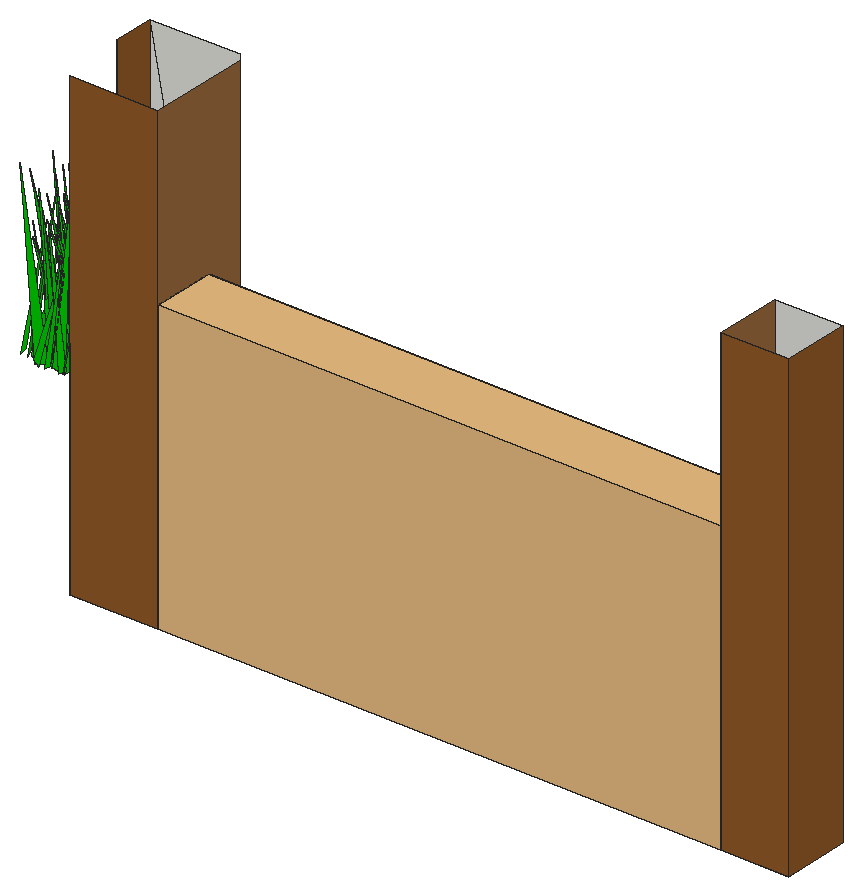
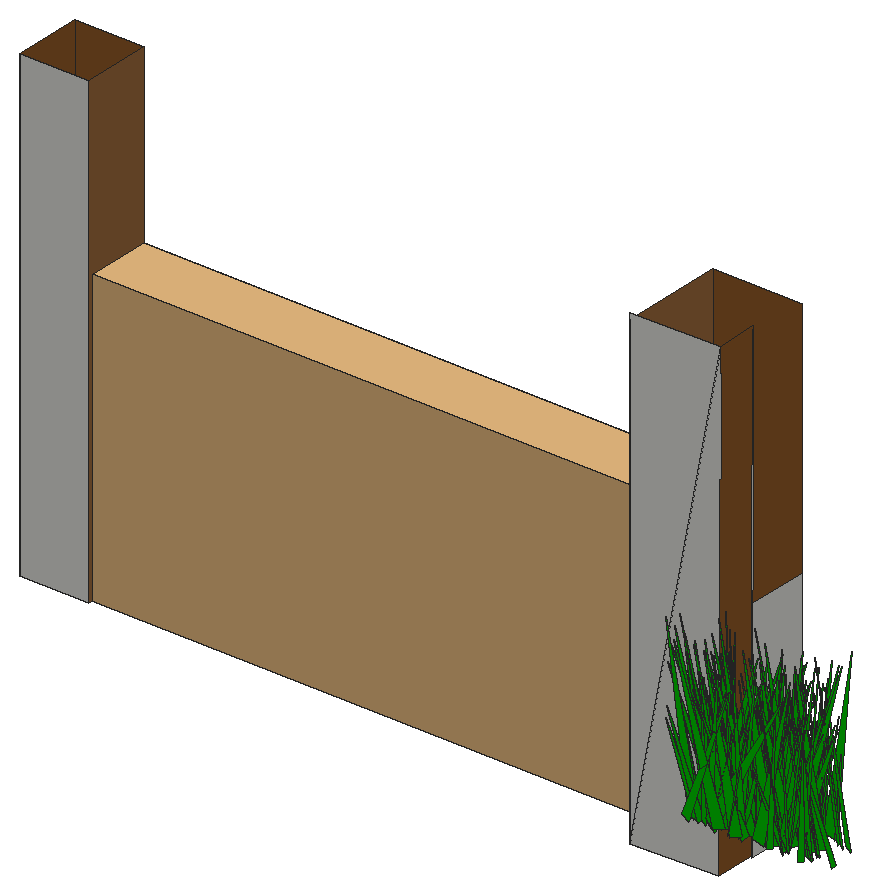
# SketchUp Ruby script. Lengths in inches.
U = 1.inch
M = Sketchup.active_model
def pt(a) = Geom::Point3d.new(a.map { |v| v * U })
def face(e, loops, mat)
  f = e.add_face(loops[0].map { |a| pt(a) })
  loops[1..].each { |l| e.add_face(l.map { |a| pt(a) }).erase! }
  f.material = f.back_material = mat if mat
  f
end
# faces: each face lists its corners as indices into pts; further lists are holes
def faces(e, pts, list, mat = nil) = list.each { |f| face(e, (f[0].is_a?(Array) ? f : [f]).map { |l| l.map { |i| pts[i] } }, mat) }
# xy, xz, yz: faces in a plane at the given z, y or x. An outline is a flat list of corners, or four numbers for a rectangle; further outlines are holes
def ring(l) = l.size == 4 ? [[l[0], l[1]], [l[2], l[1]], [l[2], l[3]], [l[0], l[3]]] : l.each_slice(2).to_a
def flat(e, list, mat, &to3) = list.each { |f| face(e, (f[0].is_a?(Array) ? f : [f]).map { |l| ring(l).map { |u, v| to3.(u, v) } }, mat) }
def xy(e, z, list, mat = nil) = flat(e, list, mat) { |x, y| [x, y, z] }
def xz(e, y, list, mat = nil) = flat(e, list, mat) { |x, z| [x, y, z] }
def yz(e, x, list, mat = nil) = flat(e, list, mat) { |y, z| [x, y, z] }
def lines(e, pts, list) = list.each { |a, b| e.add_line(pt(pts[a]), pt(pts[b])) }
# prism: a flat outline (further loops are holes) pulled along v
def prism(e, loops, v, mat = nil)
  f = face(e, loops, mat); d = Geom::Vector3d.new(v.map { |x| x * U })
  f.pushpull(f.normal.samedirection?(d) ? d.length : -d.length)
end
def box(e, o, s, mat = nil) = prism(e, [[o, [o[0] + s[0], o[1], o[2]], [o[0] + s[0], o[1] + s[1], o[2]], [o[0], o[1] + s[1], o[2]]]], [0, 0, s[2]], mat)
def at(x, y, z, deg = 0) = Geom::Transformation.translation(pt([x, y, z])) * Geom::Transformation.rotation(ORIGIN, Z_AXIS, deg.degrees)
def axes(o, x, y, z) = Geom::Transformation.new([*x, 0, *y, 0, *z, 0, *pt(o).to_a, 1])
def part(name) = M.definitions.add(name)
# library, detail: a bought-in or finely detailed component or shape, given as its bounding box
def library(name, o, s) = part(name).tap { |d| box(d.entities, o, s) }
def detail(e, o, s) = box(e.add_group.entities, o, s)
def put(e, d, t, mat = nil) = e.add_instance(d, t).tap { |i| i.material = mat if mat }
def group(e, t, mat = nil) = e.add_group.tap { |g| g.transformation = t; g.material = mat if mat }.entities
root = M.entities
M.materials.add("[Color G06]").color = [0, 204, 0]
M.materials.add("[Wood Floor Parquet]").color = [145, 89, 39]
M.materials.add("[Wood Floor]").color = [155, 105, 61]
c1 = part("fur_instance\#9")
p = [[0.8125,0,1.79],[0.67,-0.02,1.48],[0,-0.11,0],[0,0.11,0]]
faces(c1.entities,p,[[0,1,2,3]])
c2 = library("Modern+Gate+1",[0,0,0],[118.11,1.97,78.74])
xy(root,-6,[[121.48,2.125,121.48,8.54,121.67,8.29,121.67,12.5,130.61,12.75,130.61,2.125],[189.03,2.125,196.0625,9.15]])
xz(root,2.125,[[121.48,-6,130.61,42.1875],[189.03,-6,196.0625,42.0625]],"[Wood Floor Parquet]")
xz(root,9.15,[[189.03,-6,196.0625,42.0625]])
yz(root,121.48,[[2.125,-6,2.125,17.375,8.42,17.375,8.54,-6],[8.54,-6,8.54,17.375,8.42,17.375]])
yz(root,130.61,[[2.125,-6,12.75,42.1875]],"[Wood Floor]")
yz(root,189.03,[[2.125,-6,9.15,42.0625]],"[Wood Floor]")
yz(root,196.0625,[[2.125,-6,9.15,42.0625]],"[Wood Floor Parquet]")
p = [[121.67,8.29,-6],[121.48,8.54,-6],[121.48,8.42,17.375],[121.49,8.29,42.8125],[121.49,12.5,42.8125],[121.67,12.5,-6],
  [130.61,12.75,-6],[130.61,12.75,42.1875],[130.61,12.75,42.8125]]
faces(root,p,[[0,1,2,3],[5,4,6],[7,6,4,8]])
faces(root,p,[[3,4,5,0]],"[Wood Floor Parquet]")
put(root,c1,axes([107.31,16.14,4.28],[-2.23822,0.76515,2.70821],[5.77311,0.28435,1.42903],[-0.25036,-0.28356,8.74082]),"[Color G06]")
put(root,c1,axes([106.6875,16.22,4.28],[-2.84725,0.13927,0.80662],[0.78176,0.38789,-1.52926],[0.82315,0.11334,4.24241]),"[Color G06]")
put(root,c1,axes([106.91,20.07,4.28],[-5.58981,-0.32114,2.27191],[-2.05484,0.80404,1.76284],[1.84178,-0.07761,8.86202]),"[Color G06]")
put(root,c1,axes([104.89,16.85,4.28],[4.94685,-0.26614,0.07768],[-1.80121,-0.65722,-2.43716],[-0.63313,-0.20968,7.54053]),"[Color G06]")
put(root,c1,axes([103.96,19.85,4.28],[4.09901,0.34169,0.1307],[2.32033,-0.5329,-2.51227],[0.79237,-0.20708,6.68068]),"[Color G06]")
put(root,c1,axes([107.42,17.71,4.28],[-4.27879,-0.16322,0.91197],[-0.98771,0.58738,1.72486],[0.87568,-0.13501,6.40163]),"[Color G06]")
put(root,c1,axes([106.4,20,4.28],[2.27582,0.41603,0.63067],[2.88786,-0.3222,1.13794],[-0.85978,0.01899,5.49153]),"[Color G06]")
put(root,c1,axes([106.58,20.8,4.28],[-1.63991,-0.47873,0.1103],[-3.33168,0.22458,1.32609],[0.8317,-0.04431,5.5296]),"[Color G06]")
put(root,c1,axes([106,16.68,4.28],[4.25637,-0.02372,1.47172],[-0.34857,-0.59828,1.14406],[-0.93653,0.11486,6.26289]),"[Color G06]")
put(root,c1,axes([105.48,16.91,4.28],[5.82399,-0.07965,1.17242],[-0.36496,-0.7965,-2.16646],[-0.89913,-0.19262,8.47357]),"[Color G06]")
put(root,c1,axes([109.18,19.57,4.28],[-1.80742,-0.65842,1.18821],[-4.59181,0.20476,-2.5679],[-1.35702,0.18408,7.10652]),"[Color G06]")
put(root,c1,axes([106.25,19.24,4.28],[5.20739,0.12211,1.69695],[0.67046,-0.73455,1.47611],[-1.26745,0.11313,7.75282]),"[Color G06]")
put(root,c1,axes([106.3,19.02,4.28],[4.23846,0.37745,0.01663],[2.62839,-0.57459,1.77104],[-0.64692,0.13845,7.30465]),"[Color G06]")
put(root,c1,axes([108.73,19.88,4.28],[-5.82118,0.15488,1.36695],[0.79505,0.78927,-2.70996],[1.19917,0.22855,8.43237]),"[Color G06]")
put(root,c1,axes([109.85,17.24,4.28],[-4.58228,0.57529,1.07673],[4.15734,0.60686,2.27347],[-0.50588,-0.22385,8.93047]),"[Color G06]")
put(root,c1,axes([109.375,17.17,4.28],[-1.42676,-0.52227,1.51132],[-3.61847,0.12498,-2.66902],[-1.39885,0.20939,5.36261]),"[Color G06]")
put(root,c1,axes([108.07,16.57,4.28],[-4.25804,0.0751,1.83485],[-0.01705,0.56698,-2.75414],[1.34049,0.24576,5.79332]),"[Color G06]")
put(root,c1,axes([107.72,18.67,4.28],[-2.9836,-0.14143,1.40947],[-0.71691,0.42495,1.50868],[1.18496,-0.09902,4.46165]),"[Color G06]")
put(root,c1,axes([106.54,18.33,4.28],[-1.29654,0.83854,0.77196],[5.77566,0.19376,-2.50954],[1.75189,-0.01821,8.84482]),"[Color G06]")
put(root,c1,axes([108.1,16.31,4.28],[2.21507,0.47472,1.39601],[3.16348,-0.33517,1.88088],[-1.56671,-0.0056,5.77156]),"[Color G06]")
put(root,c1,axes([106.2,20.03,4.28],[4.19743,-0.1638,0.13344],[-1.13556,-0.57485,-1.27021],[-0.31341,-0.11086,6.38934]),"[Color G06]")
put(root,c1,axes([108.41,20.08,4.28],[-3.93748,-0.18116,1.02349],[-1.05205,0.53861,1.91099],[1.02468,-0.14315,5.89489]),"[Color G06]")
put(root,c1,axes([106.94,19.05,4.28],[0.48032,0.4754,1.33561],[3.45645,-0.03897,-1.18323],[0.68859,-0.136,5.00772]),"[Color G06]")
put(root,c1,axes([108.47,16.76,4.28],[1.50498,-0.80901,0.76967],[-5.64042,-0.22093,-2.041],[-1.45263,0.01969,8.72239]),"[Color G06]")
put(root,c1,axes([109.7,19.74,4.28],[-4.01086,-0.15859,0.02319],[-1.11322,0.54572,-1.35823],[-0.23335,0.12249,6.08103]),"[Color G06]")
put(root,c1,axes([109.2,19.4,4.28],[-2.44575,-0.30222,0.51286],[-2.16748,0.32156,-1.32093],[-0.34214,0.1233,4.70204]),"[Color G06]")
put(root,c1,axes([107.46,16.8125,4.28],[4.51828,0.00771,2.2813],[-0.20216,-0.65578,1.14883],[-1.51395,0.11056,6.65497]),"[Color G06]")
put(root,c1,axes([108.46,16.71,4.28],[-3.33723,-0.59604,0.26658],[-4.15397,0.45901,1.7352],[1.02283,-0.08054,7.91688]),"[Color G06]")
put(root,c1,axes([110,16.55,4.28],[-1.548,0.75045,2.8476],[5.51564,0.12556,2.89645],[-1.47316,-0.31846,7.85226]),"[Color G06]")
put(root,c1,axes([110.52,19.22,4.28],[-3.04974,-0.47656,0.10282],[-3.13603,0.38497,-2.80751],[-1.35993,0.18096,6.2436]),"[Color G06]")
put(root,c1,axes([107.57,18.48,4.28],[-1.53975,-0.45151,1.19341],[-3.04953,0.24027,1.65361],[1.34984,0.02777,5.09709]),"[Color G06]")
put(root,c1,axes([109.125,19.82,4.28],[1.73901,-0.70373,0.86131],[-4.72513,-0.25529,-2.65106],[-1.86384,-0.00939,7.52447]),"[Color G06]")
put(root,c1,axes([109.86,16.74,4.28],[-2.49989,-0.44494,0.32975],[-3.11276,0.32949,-1.64186],[-0.73505,0.11793,5.83143]),"[Color G06]")
put(root,c1,axes([107.44,18.73,4.28],[4.56358,0.38761,0.87916],[2.59044,-0.63138,1.94159],[-1.16718,0.11426,7.74663]),"[Color G06]")
put(root,c1,axes([107.63,17.43,4.28],[4.87611,0.22512,1.89335],[1.40922,-0.69839,1.43227],[-1.49173,0.07611,7.54197]),"[Color G06]")
put(root,c1,axes([106.95,15.98,4.28],[2.3343,0.36147,0.96891],[2.63093,-0.28996,-1.73202],[0.46673,-0.17335,4.91742]),"[Color G06]")
put(root,c1,axes([109.68,17.73,4.28],[-5.84303,0.30944,0.82172],[1.95745,0.78585,-2.90448],[1.18114,0.22844,8.87843]),"[Color G06]")
put(root,c1,axes([107.16,18.16,4.28],[0.54237,-0.43304,0.25884],[-2.77182,-0.05618,2.17743],[1.41091,0.0561,4.1782]),"[Color G06]")
put(root,c1,axes([107.85,19.03,4.28],[-1.67315,-0.57222,1.90362],[-3.94554,0.28008,1.92508],[1.70113,0.0868,6.33728]),"[Color G06]")
put(root,c1,axes([109.64,18.39,4.28],[-0.74934,0.42126,1.12788],[3.05594,0.07872,1.1576],[-0.59757,-0.12568,4.50558]),"[Color G06]")
put(root,c1,axes([108.07,16,4.28],[3.69626,-0.26424,0.40638],[-1.79651,-0.50727,-1.39111],[-0.66134,-0.09889,6.05015]),"[Color G06]")
put(root,c1,axes([108.39,20.2,4.28],[5.09304,-0.11864,2.20979],[-0.48141,-0.72275,-1.97914],[-1.63652,-0.15662,7.45931]),"[Color G06]")
put(root,c1,axes([109.6,16.05,4.28],[2.79981,-0.49001,2.34805],[-3.32627,-0.44433,-1.79227],[-1.93705,0.05473,6.47151]),"[Color G06]")
put(root,c1,axes([107.53,18.2,4.28],[4.05228,-0.20327,0.95642],[-1.58782,-0.53366,1.99869],[-0.11476,0.20611,6.11817]),"[Color G06]")
put(root,c1,axes([110.27,18.78,4.28],[1.79544,-0.74136,3.8567],[-5.55606,-0.33989,-1.72771],[-2.01341,0.27684,8.20684]),"[Color G06]")
put(root,c1,axes([110.0625,17.85,4.28],[-4.85266,-0.12908,2.17328],[-1.19439,0.68858,-1.25905],[1.24289,0.15772,7.2753]),"[Color G06]")
put(root,c1,axes([107.41,17.98,4.28],[1.19648,-0.43972,0.27221],[-2.77066,-0.13307,2.51032],[1.51664,0.1038,4.37122]),"[Color G06]")
put(root,c1,axes([110.39,18.76,4.28],[1.95021,0.43262,2.42784],[2.87579,-0.3458,1.9183],[-1.99838,-0.07544,5.12986]),"[Color G06]")
put(root,c1,axes([111.01,16.86,4.28],[-3.51117,-0.16643,0.60041],[-1.25725,0.47277,-1.36906],[0.07203,0.13912,5.37085]),"[Color G06]")
put(root,c1,axes([109.15,16.14,4.28],[-1.07687,0.70633,2.18414],[5.16849,0.18244,-1.08543],[1.03901,-0.17548,7.66315]),"[Color G06]")
put(root,c1,axes([111.18,20.54,4.28],[-2.05044,-0.73925,0.77051],[-5.27787,0.27162,-1.43717],[-0.71724,0.11465,8.37285]),"[Color G06]")
put(root,c1,axes([109.85,20.69,4.28],[-2.89921,-0.40686,1.35618],[-2.82722,0.42336,1.08931],[1.1589,0.01498,6.05018]),"[Color G06]")
put(root,c1,axes([108.58,20.68,4.28],[5.04342,0.12293,1.27915],[0.73734,-0.70614,1.30195],[-0.98286,0.10107,7.54049]),"[Color G06]")
put(root,c1,axes([110.9375,17.68,4.28],[-4.44335,0.07102,0.97215],[0.37042,0.6148,-1.37794],[0.73844,0.11896,6.54083]),"[Color G06]")
put(root,c1,axes([109.86,18.44,4.28],[-4.92658,-0.46949,1.35539],[-2.72073,0.65451,3.95329],[2.18073,-0.24406,7.99425]),"[Color G06]")
put(root,c1,axes([110.22,17.83,4.28],[-3.23399,0.31767,0.01701],[2.02598,0.40231,-2.68204],[1.04173,0.20376,5.26889]),"[Color G06]")
put(root,c1,axes([110.79,19.4375,4.28],[0.61727,-0.56548,1.26545],[-3.92661,-0.11791,-1.77445],[-1.32045,0.08629,5.86825]),"[Color G06]")
put(root,c1,axes([111.07,17.27,4.28],[0.46106,0.66911,1.45573],[4.71363,-0.09756,1.81673],[-1.32458,-0.11429,6.9717]),"[Color G06]")
put(root,c1,axes([110.92,18.66,4.28],[1.58525,-0.57024,0.74206],[-3.7808,-0.23086,-2.33792],[-1.63549,-0.01904,6.1239]),"[Color G06]")
put(root,c1,axes([108.65,20.41,4.28],[0.95561,0.35304,0.3803],[2.18054,-0.09409,-2.20558],[1.31142,-0.10081,3.39017]),"[Color G06]")
put(root,c1,axes([110.4,18.74,4.28],[-2.96013,-0.24864,1.17697],[-1.55222,0.42146,1.50748],[1.17897,-0.06938,4.93984]),"[Color G06]")
put(root,c1,axes([112.28,17.61,4.28],[-2.2079,-0.69049,0.46195],[-4.82067,0.28742,-2.11508],[-1.1731,0.11849,7.82215]),"[Color G06]")
put(root,c1,axes([110.71,16.72,4.28],[2.98227,0.39071,0.39782],[2.27877,-0.36694,3.23956],[-1.65184,0.19919,5.18731]),"[Color G06]")
put(root,c1,axes([112.47,18.58,4.28],[-3.98883,-0.45214,0.44555],[-3.23267,0.54204,-1.45891],[-0.38963,0.13155,7.54293]),"[Color G06]")
put(root,c1,axes([109.59,16.21,4.28],[4.20712,0.10409,1.04829],[0.56155,-0.58018,1.58369],[-0.85663,0.13088,6.18656]),"[Color G06]")
put(root,c1,axes([110.57,16.15,4.28],[-2.03863,-0.46781,0.39784],[-3.2457,0.28478,1.31659],[0.88925,-0.03303,5.7175]),"[Color G06]")
put(root,c1,axes([112.34,17.68,4.28],[-3.41621,-0.2206,0.67931],[-1.58536,0.40173,-2.82267],[-0.44259,0.26375,4.86743]),"[Color G06]")
put(root,c1,axes([110.54,17.25,4.28],[4.40092,0.31156,2.23157],[1.82955,-0.64001,2.20516],[-1.9683,0.10172,7.03931]),"[Color G06]")
put(root,c1,axes([111.36,16.33,4.28],[-2.97092,0.17488,0.14231],[1.17112,0.39708,-1.43988],[0.45854,0.11889,4.59954]),"[Color G06]")
put(root,c1,axes([111.36,19.6,4.28],[1.06334,-0.49694,2.05875],[-3.56911,-0.20035,-1.43751],[-1.36332,0.13691,5.36911]),"[Color G06]")
put(root,c1,axes([112.87,16.75,4.28],[-2.63868,0.56967,0.73763],[3.89269,0.31906,2.79904],[-1.33413,-0.19577,6.70806]),"[Color G06]")
put(root,c1,axes([110.43,17.96,4.28],[-1.56815,0.3692,1.02742],[2.54253,0.23749,-1.13503],[1.00901,-0.02463,4.45682]),"[Color G06]")
put(root,c1,axes([108.57,19.33,4.28],[2.18107,0.74092,1.74384],[5.24241,-0.23947,-2.95842],[1.45264,-0.24825,8.05831]),"[Color G06]")
put(root,c1,axes([109.15,18.24,4.28],[1.79196,0.6298,0.90057],[4.44349,-0.22156,-1.95071],[1.00843,-0.14287,6.99519]),"[Color G06]")
put(root,c1,axes([112.06,19.64,4.28],[-0.83969,-0.47527,0.17467],[-3.26391,0.10714,-1.56149],[-0.98831,0.04998,5.00844]),"[Color G06]")
put(root,c1,axes([111.92,19.59,4.28],[-1.747,0.36609,0.66426],[2.63381,0.2267,1.1205],[-0.39116,-0.10861,4.57799]),"[Color G06]")
put(root,c1,axes([108.75,16.89,4.28],[2.74419,0.42409,0.20831],[2.80908,-0.34262,-2.53244],[1.17372,-0.17152,5.5739]),"[Color G06]")
put(root,c1,axes([109.54,17.86,4.28],[2.08868,-0.69788,3.55942],[-5.4937,-0.21372,2.38728],[0.73339,0.38658,7.74558]),"[Color G06]")
put(root,c1,axes([110.76,16.5,4.28],[2.9869,0.46872,0.48005],[3.23583,-0.41442,1.50955],[-0.96482,0.06117,6.54885]),"[Color G06]")
put(root,c1,axes([110.03,19,4.28],[-0.07289,0.67882,3.48228],[5.24715,0.08491,-1.65607],[1.26224,-0.31377,7.08541]),"[Color G06]")
put(root,c1,axes([112.65,17.7,4.28],[-4.40466,0.10546,0.17552],[0.69982,0.59369,-1.75],[0.30992,0.1583,6.44611]),"[Color G06]")
put(root,c1,axes([110.31,18.9,4.28],[4.26093,0.08456,0.94185],[0.41252,-0.57972,1.81],[-0.77113,0.15709,6.17254]),"[Color G06]")
put(root,c1,axes([110.11,17.82,4.28],[4.69784,-0.1706,0.52113],[-1.04421,-0.62338,-2.41586],[-0.72658,-0.20714,6.84143]),"[Color G06]")
put(root,c1,axes([114.08,17.28,4.28],[-2.74277,-0.73578,1.6827],[-5.12249,0.29985,-3.58942],[-1.69375,0.28464,8.13081]),"[Color G06]")
put(root,c1,axes([112.05,18.1,4.28],[1.7613,0.4092,0.0381],[2.53786,-0.21448,2.54841],[-1.47339,0.11972,4.43507]),"[Color G06]")
put(root,c1,axes([109.9375,20.27,4.28],[1.18857,-0.81084,1.5956],[-5.76813,-0.12576,2.25615],[1.29595,0.18389,8.5785]),"[Color G06]")
put(root,c1,axes([110.54,17.9,4.28],[1.40951,-0.47217,0.79495],[-3.375,-0.1772,1.27643],[0.59791,0.11284,5.33095]),"[Color G06]")
put(root,c1,axes([113.125,20.08,4.28],[-4.32853,0.10501,1.31017],[1.03156,0.56471,2.41336],[0.52098,-0.2457,6.1069]),"[Color G06]")
put(root,c1,axes([112.81,17.23,4.28],[2.60179,0.57479,3.08226],[4.02763,-0.44409,1.9191],[-2.24092,-0.13082,7.02784]),"[Color G06]")
put(root,c1,axes([114,16.03,4.28],[-2.42354,0.71572,0.46214],[4.98682,0.31555,2.27825],[-1.25327,-0.12845,8.17156]),"[Color G06]")
put(root,c1,axes([111.74,19.68,4.28],[3.43036,-0.25573,1.39293],[-1.62779,-0.49195,-1.42077],[-1.25785,-0.0608,5.63733]),"[Color G06]")
put(root,c1,axes([112.58,19.5,4.28],[-3.63962,-0.31987,0.2067],[-2.06347,0.4708,2.5325],[1.01148,-0.19055,5.91019]),"[Color G06]")
put(root,c1,axes([111.46,16.68,4.28],[2.63126,0.21517,0.30303],[1.45467,-0.35977,1.13151],[-0.55325,0.07741,4.4163]),"[Color G06]")
put(root,c1,axes([112.5625,18.62,4.28],[-3.65829,-0.39515,0.86318],[-2.68349,0.51223,1.53294],[1.0782,-0.06586,6.74401]),"[Color G06]")
put(root,c1,axes([112.21,17.91,4.28],[2.88314,0.13717,1.68111],[0.7161,-0.42601,1.24969],[-1.31148,0.06893,4.37808]),"[Color G06]")
put(root,c1,axes([115.96,20.66,4.28],[-4.01121,0.62048,0.66511],[3.87034,0.43995,4.99133],[-2.23997,-0.35094,7.43325]),"[Color G06]")
put(root,c1,axes([111.58,18.53,4.28],[-1.05759,-0.43714,1.62122],[-3.02819,0.19204,1.53583],[1.35429,0.08803,4.70016]),"[Color G06]")
put(root,c1,axes([110.94,16.15,4.28],[4.48965,-0.07633,0.29865],[-0.40305,-0.56314,-2.99851],[-0.42081,-0.27496,6.05836]),"[Color G06]")
put(root,c1,axes([113.41,20.04,4.28],[-5.22,0.32562,1.03794],[2.09813,0.71726,-2.27854],[1.2381,0.15737,8.23738]),"[Color G06]")
put(root,c1,axes([111.45,16.81,4.28],[4.6935,0.02729,1.44758],[-0.0453,-0.64895,1.73366],[-0.9871,0.15956,6.80347]),"[Color G06]")
put(root,c1,axes([112.52,15.97,4.28],[2.41668,0.19032,0.86524],[1.21917,-0.34296,1.05987],[-0.84359,0.04958,4.01045]),"[Color G06]")
put(root,c1,axes([112.83,16.24,4.28],[-3.54038,-0.52781,0.10039],[-3.4497,0.45509,3.10442],[1.55913,-0.19161,7.09673]),"[Color G06]")
put(root,c1,axes([113.99,20.78,4.28],[-4.30977,0.06843,0.86372],[0.30775,0.58299,-1.87592],[0.69289,0.16671,6.20555]),"[Color G06]")
put(root,c1,axes([110.56,18.53,4.28],[2.0276,0.45964,0.92146],[2.81868,-0.17918,-3.58712],[1.81668,-0.23501,4.53717]),"[Color G06]")
put(root,c1,axes([113.93,16.67,4.28],[0.157,-0.72532,1.5759],[-5.19731,-0.0508,-1.52913],[-1.07463,0.13971,7.62569]),"[Color G06]")
put(root,c1,axes([112.89,20.47,4.28],[-4.36634,0.47418,1.8703],[2.86835,0.61929,-3.07874],[2.21403,0.13283,7.67706]),"[Color G06]")
put(root,c1,axes([113.31,15.89,4.28],[-3.27802,-0.60617,0.78096],[-4.19259,0.46082,1.77877],[1.26162,-0.04361,7.94031]),"[Color G06]")
put(root,c1,axes([113.25,17.17,4.28],[-2.53208,0.46167,0.98533],[3.22338,0.36479,-1.13195],[1.00291,-0.00685,6.12577]),"[Color G06]")
put(root,c1,axes([112.28,19.47,4.28],[4.01499,-0.38445,0.36378],[-2.68494,-0.55554,-1.2506],[-0.67192,-0.07738,7.17101]),"[Color G06]")
put(root,c1,axes([111.58,15.92,4.28],[5.5387,-0.23758,1.37739],[-1.85936,-0.76121,1.61846],[-0.54296,0.18326,8.50821]),"[Color G06]")
put(root,c1,axes([113.7,18.66,4.28],[3.39561,0.53498,2.90105],[3.86396,-0.53097,1.14545],[-1.88571,-0.12466,7.57104]),"[Color G06]")
put(root,c1,axes([116.05,17.92,4.28],[-6.05157,0.14883,0.07547],[1.05618,0.82709,1.81075],[-0.16168,-0.16758,9.00383]),"[Color G06]")
put(root,c1,axes([116.1875,19.84,4.28],[-4.94525,0.3787,0.27581],[2.66685,0.66337,2.1771],[-0.54529,-0.19011,8.14632]),"[Color G06]")
put(root,c1,axes([112.4,17.5,4.28],[4.56714,0.03244,0.94171],[0.34631,-0.63115,-1.254],[-0.5755,-0.12235,6.71875]),"[Color G06]")
put(root,c1,axes([113.2,19.04,4.28],[3.20773,-0.263,0.36182],[-1.72696,-0.43064,-1.75924],[-0.79584,-0.12556,5.2759]),"[Color G06]")
put(root,c1,axes([114.36,17.61,4.28],[-3.5603,-0.3779,0.40701],[-2.54002,0.48324,1.90995],[0.98311,-0.12002,6.40868]),"[Color G06]")
put(root,c1,axes([113.71,17.39,4.28],[-2.53993,0.34915,0.44462],[2.16722,0.33239,-2.32984],[1.28871,0.12915,4.79437]),"[Color G06]")
put(root,c1,axes([115.26,19.09,4.28],[1.57889,0.48146,0.35069],[2.85935,-0.20175,3.06287],[-1.94941,0.09402,4.77659]),"[Color G06]")
put(root,c1,axes([115.55,18.58,4.28],[-0.67288,0.52113,1.51537],[3.67749,0.04106,2.02543],[-1.21263,-0.16464,5.30155]),"[Color G06]")
put(root,c1,axes([116,18.41,4.28],[-1.54522,0.6201,1.64759],[4.41628,0.15842,2.4024],[-1.21934,-0.21204,6.61321]),"[Color G06]")
put(root,c1,axes([114.2,20.16,4.28],[3.72641,0.39027,1.20353],[2.45093,-0.51876,2.37287],[-1.57294,0.11625,6.54859]),"[Color G06]")
put(root,c1,axes([115.87,16.68,4.28],[-0.71813,0.70906,1.57639],[5.03595,0.05884,2.08429],[-1.26774,-0.16792,7.38664]),"[Color G06]")
put(root,c1,axes([112.3,20.02,4.28],[3.73954,-0.60423,0.40657],[-4.27634,-0.50397,1.82134],[0.74995,0.13921,8.35822]),"[Color G06]")
put(root,c1,axes([112.55,19.7,4.28],[1.96043,0.56962,0.17715],[3.86095,-0.25216,-2.29943],[1.33929,-0.10687,6.36956]),"[Color G06]")
put(root,c1,axes([114.85,19.69,4.28],[-2.906,0.17025,1.00614],[0.91576,0.39673,-1.80326],[1.05124,0.12502,4.35217]),"[Color G06]")
put(root,c1,axes([116.99,19.09,4.28],[-1.86575,-0.7668,1.22571],[-5.32988,0.21236,-2.86117],[-1.58208,0.18887,8.19352]),"[Color G06]")
put(root,c1,axes([116.43,19.83,4.28],[-4.67554,0.09441,0.05818],[0.57995,0.57628,-3.31022],[0.35143,0.30498,6.23679]),"[Color G06]")
put(root,c1,axes([112.85,19.07,4.28],[2.48331,0.76952,1.43186],[5.47602,-0.30287,-2.51594],[1.1766,-0.21455,8.68737]),"[Color G06]")
put(root,c1,axes([113.16,20.96,4.28],[1.31689,-0.775,1.43323],[-5.47349,-0.14252,2.38112],[1.35963,0.17689,8.19757]),"[Color G06]")
put(root,c1,axes([115.39,17.02,4.28],[1.39546,0.32241,1.20755],[2.19433,-0.22218,1.15005],[-1.08783,-0.03459,3.86886]),"[Color G06]")
put(root,c1,axes([113.59,16.5,4.28],[4.01861,0.21308,1.36406],[1.76375,-0.51892,-2.29514],[-0.23885,-0.24687,6.00177]),"[Color G06]")
put(root,c1,axes([115.07,19.98,4.28],[-3.25987,-0.08054,1.93258],[0.06989,0.44282,2.38342],[1.41449,-0.20751,4.33614]),"[Color G06]")
put(root,c1,axes([115.55,16.33,4.28],[1.27694,-0.34682,1.39735],[-2.38627,-0.21331,-1.21093],[-1.16871,0.05659,3.99925]),"[Color G06]")
put(root,c1,axes([114.36,20.23,4.28],[5.14426,0.22998,1.95673],[1.38686,-0.73267,1.74779],[-1.58451,0.10537,7.88249]),"[Color G06]")
put(root,c1,axes([112.42,20.64,4.28],[4.12729,-0.36581,0.12987],[-2.40142,-0.51716,3.13599],[1.05947,0.25284,6.60216]),"[Color G06]")
put(root,c1,axes([116.4,16.07,4.28],[-3.13881,-0.02475,0.0605],[-0.17194,0.37091,-2.49224],[-0.05991,0.23245,3.98325]),"[Color G06]")
put(root,c1,axes([116.36,17.62,4.28],[-2.04155,-0.59552,1.29543],[-4.34539,0.26819,-1.13451],[-0.32725,0.15405,6.98304]),"[Color G06]")
put(root,c1,axes([113.62,20.2,4.28],[4.09605,0.23384,0.75366],[1.75108,-0.54585,-1.80289],[0.011,-0.18231,6.3646]),"[Color G06]")
put(root,c1,axes([113.46,17.78,4.28],[5.39455,0.18326,1.62532],[1.68338,-0.65321,-4.01991],[-0.27561,-0.40273,7.25969]),"[Color G06]")
put(root,c1,axes([117.01,17.39,4.28],[-1.00203,-0.46107,1.24142],[-3.15326,0.07945,-2.29551],[-1.29597,0.16318,4.6254]),"[Color G06]")
put(root,c1,axes([114.67,20.24,4.28],[0.64811,-0.35102,1.20072],[-2.55685,-0.05421,1.2624],[0.66672,0.13334,3.67409]),"[Color G06]")
put(root,c1,axes([116.11,18.82,4.28],[0.89428,-0.40152,0.36692],[-2.71209,-0.12898,-1.44916],[-0.99799,-0.00928,4.26694]),"[Color G06]")
put(root,c1,axes([116.31,20.51,4.28],[2.94359,0.60465,1.60727],[3.92452,-0.43579,2.77787],[-2.13457,0.0326,7.32371]),"[Color G06]")
put(root,c1,axes([116.53,17.05,4.28],[0.00065,-0.47035,0.3525],[-3.22667,-0.00992,-1.50672],[-1.01063,0.03136,4.81076]),"[Color G06]")
put(root,c1,axes([116.36,18.48,4.28],[-5.70877,0.02574,2.70192],[-0.31649,0.80432,-2.37378],[1.78944,0.22436,8.19996]),"[Color G06]")
put(root,c1,axes([116.07,18.99,4.28],[-2.88795,-0.24321,0.39798],[-1.53974,0.3822,1.87269],[0.86141,-0.13221,4.68166]),"[Color G06]")
put(root,c1,axes([116.4375,18.4375,4.28],[0.07872,0.42749,0.03049],[2.94692,-0.01134,1.26286],[-0.84521,0.00029,4.40596]),"[Color G06]")
put(root,c1,axes([116.05,16.9375,4.28],[-3.17394,-0.01233,1.79861],[-0.44838,0.45046,-1.41277],[1.12027,0.14537,4.53036]),"[Color G06]")
put(root,c1,axes([115.66,18.89,4.28],[3.53347,0.07208,2.62829],[1.08772,-0.5111,-1.65635],[-1.47531,-0.20419,5.07373]),"[Color G06]")
put(root,c1,axes([115.16,19.62,4.28],[3.2516,-0.13888,1.54034],[-1.22239,-0.45476,1.0538],[-0.74825,0.13941,4.97216]),"[Color G06]")
put(root,c1,axes([118.25,16.17,4.28],[-4.95997,-0.15097,0.15009],[-1.01267,0.61761,-3.38893],[-0.39587,0.31165,6.78871]),"[Color G06]")
put(root,c1,axes([116.33,19.61,4.28],[-4.73203,-0.10706,2.82071],[-1.1763,0.68691,-1.41306],[1.66363,0.18118,7.02412]),"[Color G06]")
put(root,c1,axes([115.95,17.85,4.28],[5.11845,0.00015,3.55147],[0.42486,-0.77429,-1.36389],[-2.33795,-0.14037,7.52733]),"[Color G06]")
put(root,c1,axes([114.58,20.43,4.28],[3.6969,-0.41136,1.27398],[-3.06785,-0.50273,1.23847],[-0.13081,0.16477,6.95942]),"[Color G06]")
put(root,c1,axes([115.98,17.75,4.28],[2.94677,0.15717,1.30698],[0.56945,-0.38619,2.46695],[-1.30798,0.18596,4.01852]),"[Color G06]")
put(root,c1,axes([115.08,17.98,4.28],[2.995,-0.12923,0.87892],[-1.06228,-0.40125,1.30833],[-0.27616,0.14192,4.49929]),"[Color G06]")
put(root,c1,axes([118.25,21,4.28],[-3.25718,-0.52459,0.09224],[-3.64905,0.43767,-1.88999],[-0.91703,0.12173,7.19305]),"[Color G06]")
put(root,c1,axes([116.61,19.41,4.28],[3.3187,0.49082,0.86746],[2.93069,-0.43815,3.4337],[-2.03398,0.16953,6.36286]),"[Color G06]")
put(root,c1,axes([115.01,17.57,4.28],[3.39148,-0.01369,0.37391],[-0.03673,-0.46109,-1.19497],[-0.26623,-0.11077,4.92812]),"[Color G06]")
put(root,c1,axes([116.09,17.38,4.28],[5.39021,0.15218,3.22235],[0.49591,-0.78895,2.4273],[-2.36508,0.18141,7.85295]),"[Color G06]")
put(root,c1,axes([116.19,19.41,4.28],[-1.96064,0.45301,0.01352],[3.13053,0.26385,-1.50773],[0.86821,0.07165,5.46703]),"[Color G06]")
put(root,c1,axes([117.76,20.6,4.28],[-0.24296,-0.64376,1.16903],[-4.39409,-0.00639,-2.44382],[-1.61762,0.11403,6.46277]),"[Color G06]")
put(root,c1,axes([117.08,18.375,4.28],[0.07673,0.53708,0.53972],[3.7457,-0.0229,1.42835],[-0.96666,-0.04611,5.57755]),"[Color G06]")
put(root,c1,axes([115.53,19.05,4.28],[3.17803,-0.39264,0.12777],[-2.74452,-0.43561,-1.28949],[-0.63492,-0.08233,6.21349]),"[Color G06]")
put(root,c1,axes([116.16,17.78,4.28],[2.86421,0.1996,0.88167],[1.04611,-0.37705,2.21438],[-1.14127,0.15532,4.24243]),"[Color G06]")
put(root,c1,axes([115.71,18.2,4.28],[-1.57995,-0.62656,2.14662],[-4.46593,0.26669,1.5999],[1.51903,0.13239,6.9364]),"[Color G06]")
put(root,c1,axes([115.14,17.27,4.28],[3.07264,-0.67205,2.20684],[-5.03834,-0.40232,1.59559],[0.14994,0.25322,8.39207]),"[Color G06]")
put(root,c1,axes([114.74,19.79,4.28],[4.56095,0.09565,0.26078],[0.70709,-0.62264,-1.39066],[-0.03052,-0.13194,6.75159]),"[Color G06]")
put(root,c1,axes([117.3,16.27,4.28],[1.47318,-0.32978,0.84036],[-2.1218,-0.21918,-1.57234],[-1.18624,-0.0175,3.85604]),"[Color G06]")
put(root,c1,axes([116.62,19.7,4.28],[3.63406,-0.23149,2.80471],[-2.14716,-0.52533,1.23358],[-1.29121,0.22205,5.84243]),"[Color G06]")
put(root,c1,axes([116.66,20.67,4.28],[3.89049,-0.29485,1.52478],[-1.84381,-0.55419,-1.80195],[-1.45333,-0.08622,6.36787]),"[Color G06]")
put(root,c1,axes([116.73,19.7,4.28],[3.42868,-0.425,0.83066],[-2.80555,-0.47498,-2.04945],[-1.31409,-0.09482,6.54284]),"[Color G06]")
put(root,c1,axes([117.31,19.93,4.28],[-2.18087,0.4448,0.00541],[3.13437,0.29894,-1.06827],[0.59205,0.05584,5.67547]),"[Color G06]")
put(root,c1,axes([113.64,20.04,4.28],[3.75569,0.67638,0.506],[4.36866,-0.44321,-4.37263],[2.13463,-0.28296,8.05862]),"[Color G06]")
put(root,c1,axes([115.09,20.74,4.28],[1.50097,0.83584,0.38351],[5.7747,-0.19127,-2.59651],[1.62689,-0.09221,8.86256]),"[Color G06]")
put(root,c1,axes([115.39,18.95,4.28],[2.93523,-0.61323,1.31069],[-4.41519,-0.36967,2.21812],[0.784,0.21408,7.5845]),"[Color G06]")
put(root,c1,axes([115.33,19.6875,4.28],[5.77069,-0.12995,0.88043],[-1.02317,-0.79428,1.51304],[-0.41055,0.15297,8.60444]),"[Color G06]")
put(root,c1,axes([117.3,16.11,4.28],[-5.4851,0.0121,4.21641],[-0.83685,0.81416,-2.70011],[2.69556,0.27737,7.74155]),"[Color G06]")
put(root,c1,axes([116.54,17.57,4.28],[-3.4758,0.48592,3.23148],[3.01422,0.5707,-2.61616],[2.78072,-0.01123,6.87508]),"[Color G06]")
put(root,c1,axes([116.1875,19.93,4.28],[1.98678,-0.62344,2.52597],[-4.72875,-0.21925,2.0919],[0.69558,0.29022,7.00646]),"[Color G06]")
put(root,c1,axes([115.64,16.17,4.28],[3.11016,0.48566,0.10421],[3.38348,-0.41806,-1.75047],[0.82873,-0.11582,6.7556]),"[Color G06]")
put(root,c1,axes([117.73,15.92,4.28],[3.59173,-0.34318,1.96669],[-2.35014,-0.53323,-1.10134],[-1.50498,0.01367,6.41345]),"[Color G06]")
put(root,c1,axes([116.31,19.96,4.28],[1.85226,0.7809,1.9637],[5.62212,-0.20508,-2.47701],[1.21609,-0.24129,8.46051]),"[Color G06]")
put(root,c1,axes([116.875,19.55,4.28],[-1.78078,0.68071,3.40556],[4.89305,0.34438,-2.19233],[2.25384,-0.20982,7.45028]),"[Color G06]")
put(root,c1,axes([117.28,18.99,4.28],[0.17654,-0.41039,0.56656],[-2.7977,-0.00537,1.50023],[0.98889,0.05806,4.1432]),"[Color G06]")
put(root,c1,axes([117.96,16.77,4.28],[2.86855,0.04619,1.14902],[0.12698,-0.40226,1.14945],[-0.82743,0.0984,4.15987]),"[Color G06]")
put(root,c1,axes([117.03,20.64,4.28],[1.77214,0.43227,1.06205],[2.98435,-0.18682,-2.38836],[1.09915,-0.18969,4.77242]),"[Color G06]")
put(root,c1,axes([116.25,19.28,4.28],[3.27443,0.53358,0.03033],[3.58529,-0.42651,-2.6546],[1.33716,-0.16305,7.04339]),"[Color G06]")
put(root,c1,axes([117.59,17.8,4.28],[0.77946,-0.71844,0.54004],[-5.0421,-0.09481,1.7666],[1.11888,0.07324,7.58479]),"[Color G06]")
put(root,c1,axes([117.5625,20.46,4.28],[1.03242,0.42824,0.55742],[2.82653,-0.10829,-2.13678],[1.25746,-0.10819,4.3454]),"[Color G06]")
put(root,c1,axes([118.0625,19.35,4.28],[4.09491,0.30204,0.08955],[2.08521,-0.55415,1.71894],[-0.58911,0.138,6.7068]),"[Color G06]")
put(root,c1,axes([117.79,20.49,4.28],[3.23013,0.67435,2.82926],[5.19088,-0.40989,-2.01508],[0.15626,-0.32335,8.45486]),"[Color G06]")
put(root,c1,axes([117.23,18.21,4.28],[5.97223,0.08587,0.90229],[0.7289,-0.81744,-1.84039],[-0.46082,-0.18012,8.78251]),"[Color G06]")
put(root,c1,axes([118.04,19.43,4.28],[3.95828,0.30034,1.47336],[2.36446,-0.51697,-2.08368],[-0.14134,-0.23728,6.40458]),"[Color G06]")
put(root,c2,axes([130.61,8.74,-6],[0.49466,0,0],[0,-3.36184,0],[0,0,0.3822]))
